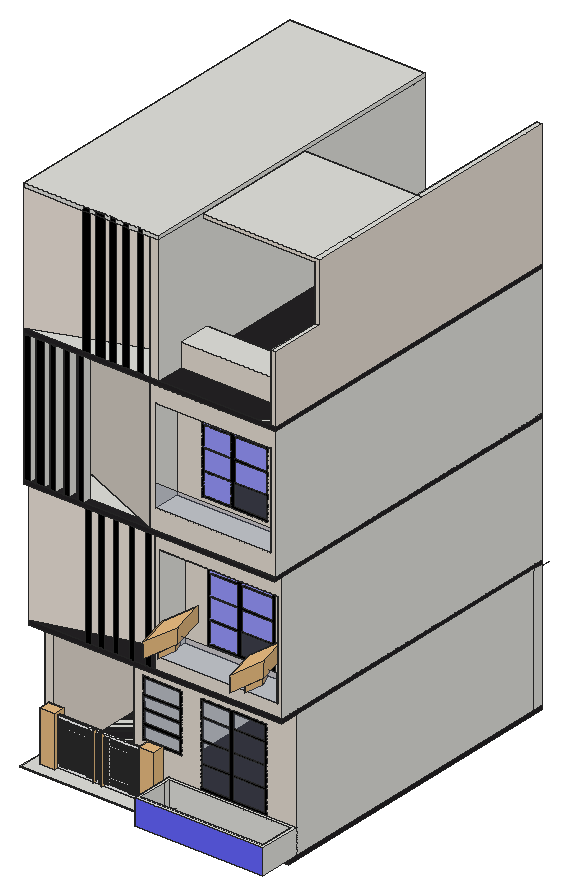
# SketchUp Ruby script. Lengths in inches.
U = 1.inch
M = Sketchup.active_model
def pt(a) = Geom::Point3d.new(a.map { |v| v * U })
def face(e, loops, mat)
  f = e.add_face(loops[0].map { |a| pt(a) })
  loops[1..].each { |l| e.add_face(l.map { |a| pt(a) }).erase! }
  f.material = f.back_material = mat if mat
  f
end
# faces: each face lists its corners as indices into pts; further lists are holes
def faces(e, pts, list, mat = nil) = list.each { |f| face(e, (f[0].is_a?(Array) ? f : [f]).map { |l| l.map { |i| pts[i] } }, mat) }
# xy, xz, yz: faces in a plane at the given z, y or x. An outline is a flat list of corners, or four numbers for a rectangle; further outlines are holes
def ring(l) = l.size == 4 ? [[l[0], l[1]], [l[2], l[1]], [l[2], l[3]], [l[0], l[3]]] : l.each_slice(2).to_a
def flat(e, list, mat, &to3) = list.each { |f| face(e, (f[0].is_a?(Array) ? f : [f]).map { |l| ring(l).map { |u, v| to3.(u, v) } }, mat) }
def xy(e, z, list, mat = nil) = flat(e, list, mat) { |x, y| [x, y, z] }
def xz(e, y, list, mat = nil) = flat(e, list, mat) { |x, z| [x, y, z] }
def yz(e, x, list, mat = nil) = flat(e, list, mat) { |y, z| [x, y, z] }
def lines(e, pts, list) = list.each { |a, b| e.add_line(pt(pts[a]), pt(pts[b])) }
# prism: a flat outline (further loops are holes) pulled along v
def prism(e, loops, v, mat = nil)
  f = face(e, loops, mat); d = Geom::Vector3d.new(v.map { |x| x * U })
  f.pushpull(f.normal.samedirection?(d) ? d.length : -d.length)
end
def box(e, o, s, mat = nil) = prism(e, [[o, [o[0] + s[0], o[1], o[2]], [o[0] + s[0], o[1] + s[1], o[2]], [o[0], o[1] + s[1], o[2]]]], [0, 0, s[2]], mat)
def at(x, y, z, deg = 0) = Geom::Transformation.translation(pt([x, y, z])) * Geom::Transformation.rotation(ORIGIN, Z_AXIS, deg.degrees)
def axes(o, x, y, z) = Geom::Transformation.new([*x, 0, *y, 0, *z, 0, *pt(o).to_a, 1])
def part(name) = M.definitions.add(name)
# library, detail: a bought-in or finely detailed component or shape, given as its bounding box
def library(name, o, s) = part(name).tap { |d| box(d.entities, o, s) }
def detail(e, o, s) = box(e.add_group.entities, o, s)
def put(e, d, t, mat = nil) = e.add_instance(d, t).tap { |i| i.material = mat if mat }
def group(e, t, mat = nil) = e.add_group.tap { |g| g.transformation = t; g.material = mat if mat }.entities
root = M.entities
M.materials.add("02 - Default").color = [196, 209, 187]
M.materials.add("02 - DefaultW").color = [91, 118, 29]
M.materials.add("04 - Default").color = [38, 38, 38]
M.materials.add("04 - DefaultW").color = [92, 55, 26]
M.materials.add("06 - Default").color = [255, 255, 255]
M.materials.add("07 - Default").color = [92, 55, 26]
M.materials.add("10 - Default").color = [62, 56, 39]
M.materials.add("Glass_Sky Reflection_01").color = [126, 138, 183]
M.materials["Glass_Sky Reflection_01"].alpha = 0.25
M.materials.add("I02_Moonlit_Azure").color = [153, 153, 255]
M.materials.add("I03_Bluebell_Mist").color = [101, 101, 255]
M.materials.add("M09_Shadow_Night").color = [0, 0, 0]
M.materials.add("Marble_01_1K").color = [230, 221, 211]
M.materials.add("Marble_07_1K").color = [36, 34, 36]
M.materials.add("Plywood_01_1K").color = [125, 96, 64]
M.materials.add("[Color_000]").color = [255, 255, 255]
M.materials.add("[Color_C20]").color = [102, 91, 81]
c1 = part("Horizontal gate slat")
xy(c1.entities,0,[[0.39,114.16,6.3,114.17]])
xy(c1.entities,0,[[0.39,0,6.3,114.16]],"[Color_C20]")
xy(c1.entities,0.39,[[0.39,0,0.79,114.17],[0.98,0,2.07,114.17],[2.36,0,3.2,114.17],[3.59,0,4.37,114.17],[4.56,0,5.71,114.17],
  [5.91,0,6.3,114.17]],"[Color_C20]")
xy(c1.entities,0.79,[[0.39,0,0.79,114.17],[0.98,0,2.07,114.17],[2.36,0,3.2,114.17],[3.59,0,4.37,114.17],[4.56,0,5.71,114.17],
  [5.91,0,6.3,114.17]],"[Color_C20]")
xy(c1.entities,0.99,[[1.13,0,1.21,114.16],[1.87,0,1.94,114.16],[2.61,0,2.68,114.16],[3.35,0,3.42,114.16],[4.08,0,4.16,114.16],
  [4.82,0,4.9,114.16],[5.5625,0,5.63,114.16],[6.3,0,6.37,114.16]],"[Color_C20]")
xy(c1.entities,1.18,[[0.39,114.16,3.35,114.17],[3.35,114.16,6.3,114.17]])
xy(c1.entities,1.18,[[0.39,0,1.13,114.16],[1.21,0,1.87,114.16],[1.94,0,2.61,114.16],[2.68,0,3.35,114.16],[3.42,0,4.08,114.16],
  [4.16,0,4.82,114.16],[4.9,0,5.5625,114.16],[5.63,0,6.3,114.16]],"[Color_C20]")
xz(c1.entities,0,[[[0.39,0,6.3,0,6.3,0.39,5.91,0.39,5.91,0.79,6.3,0.79,6.3,1.18,5.63,1.18,5.63,0.99,5.5625,0.99,5.5625,1.18,4.9,1.18,4.9,0.99,4.82,0.99,4.82,1.18,4.16,1.18,4.16,0.99,4.08,0.99,4.08,1.18,3.42,1.18,3.42,0.99,3.35,0.99,3.35,1.18,2.68,1.18,2.68,0.99,2.61,0.99,2.61,1.18,1.94,1.18,1.94,0.99,1.87,0.99,1.87,1.18,1.21,1.18,1.21,0.99,1.13,0.99,1.13,1.18,0.39,1.18,0.39,0.79,0.79,0.79,0.79,0.39,0.39,0.39],[4.56,0.39,5.71,0.79],[0.98,0.39,2.07,0.79],[2.36,0.39,3.2,0.79],[3.59,0.39,4.37,0.79]],[6.3,0.99,6.37,1.18]],"[Color_C20]")
xz(c1.entities,114.16,[[1.13,0.99,1.21,1.18],[1.87,0.99,1.94,1.18],[2.61,0.99,2.68,1.18],[3.35,0.99,3.42,1.18],[4.08,0.99,4.16,1.18],
  [4.82,0.99,4.9,1.18],[5.5625,0.99,5.63,1.18]],"[Color_C20]")
xz(c1.entities,114.17,[[[0.39,0,0.39,0.39,0.79,0.39,0.79,0.79,0.39,0.79,0.39,1.18,6.3,1.18,6.3,0.79,5.91,0.79,5.91,0.39,6.3,0.39,6.3,0],[4.56,0.39,5.71,0.79],[0.98,0.39,2.07,0.79],[2.36,0.39,3.2,0.79],[3.59,0.39,4.37,0.79]]],"[Color_C20]")
yz(c1.entities,0.39,[[114.16,0,114.17,0.39],[114.16,0.79,114.17,1.18]])
yz(c1.entities,0.39,[[0,0,114.16,0.39],[0,0.79,114.16,1.18]],"[Color_C20]")
yz(c1.entities,0.79,[[0,0.39,114.17,0.79]],"[Color_C20]")
yz(c1.entities,0.98,[[0,0.39,114.17,0.79]],"[Color_C20]")
yz(c1.entities,1.13,[[0,0.99,114.16,1.18]],"[Color_C20]")
yz(c1.entities,1.21,[[0,0.99,114.16,1.18]],"[Color_C20]")
yz(c1.entities,1.87,[[0,0.99,114.16,1.18]],"[Color_C20]")
yz(c1.entities,1.94,[[0,0.99,114.16,1.18]],"[Color_C20]")
yz(c1.entities,2.07,[[0,0.39,114.17,0.79]],"[Color_C20]")
yz(c1.entities,2.36,[[0,0.39,114.17,0.79]],"[Color_C20]")
yz(c1.entities,2.61,[[0,0.99,114.16,1.18]],"[Color_C20]")
yz(c1.entities,2.68,[[0,0.99,114.16,1.18]],"[Color_C20]")
yz(c1.entities,3.2,[[0,0.39,114.17,0.79]],"[Color_C20]")
yz(c1.entities,3.35,[[0,0.99,114.16,1.18]],"[Color_C20]")
yz(c1.entities,3.42,[[0,0.99,114.16,1.18]],"[Color_C20]")
yz(c1.entities,3.59,[[0,0.39,114.17,0.79]],"[Color_C20]")
yz(c1.entities,4.08,[[0,0.99,114.16,1.18]],"[Color_C20]")
yz(c1.entities,4.16,[[0,0.99,114.16,1.18]],"[Color_C20]")
yz(c1.entities,4.37,[[0,0.39,114.17,0.79]],"[Color_C20]")
yz(c1.entities,4.56,[[0,0.39,114.17,0.79]],"[Color_C20]")
yz(c1.entities,4.82,[[0,0.99,114.16,1.18]],"[Color_C20]")
yz(c1.entities,4.9,[[0,0.99,114.16,1.18]],"[Color_C20]")
yz(c1.entities,5.5625,[[0,0.99,114.16,1.18]],"[Color_C20]")
yz(c1.entities,5.63,[[0,0.99,114.16,1.18]],"[Color_C20]")
yz(c1.entities,5.71,[[0,0.39,114.17,0.79]],"[Color_C20]")
yz(c1.entities,5.91,[[0,0.39,114.17,0.79]],"[Color_C20]")
yz(c1.entities,6.3,[[114.16,0,114.17,0.39],[114.16,0.79,114.17,1.18]])
yz(c1.entities,6.3,[[0,0,114.16,0.39],[0,0.79,114.16,0.99],[0,0.99,114.16,1.18]],"[Color_C20]")
yz(c1.entities,6.37,[[0,0.99,114.16,1.18]],"[Color_C20]")
p = [[0,0,0],[0.39,0,0]]
lines(c1.entities,p,[[0,1]])
c2 = part("Vertical gate panel")
put(c2.entities,c1,axes([0,1.18,0],[3.67755,0,0],[0,0,2.40086],[0,-1,0]))
put(c2.entities,c1,axes([21.72,1.18,0],[3.67755,0,0],[0,0,2.40086],[0,-1,0]))
c3 = library("Gate pull handle",[-0.01,0,0],[1.26,2.875,48])
c4 = part("Slatted gate assembly")
xy(c4.entities,0,[[553.15,18.86,552.64,18.92,552.18,19.1,551.78,19.39,551.47,19.76,551.27,20.2,551.21,20.67,551.27,21.13,551.47,21.57,551.78,21.94,552.18,22.23,552.64,22.41,553.15,22.47,553.65,22.41,554.11,22.23,554.52,21.94,554.82,21.57,555.02,21.13,555.08,20.67,555.02,20.2,554.82,19.76,554.52,19.39,554.11,19.1,553.65,18.92],[12.73,19.29,12.23,19.35,11.76,19.55,11.36,19.85,11.05,20.25,10.86,20.72,10.79,21.22,10.86,21.72,11.05,22.19,11.36,22.59,11.76,22.9,12.23,23.09,12.73,23.16,13.23,23.09,13.7,22.9,14.1,22.59,14.41,22.19,14.6,21.72,14.67,21.22,14.6,20.72,14.41,20.25,14.1,19.85,13.7,19.55,13.23,19.35]])
xy(c4.entities,5.93,[[[4.54,12.88,282.375,27.63],[12.73,19.29,13.23,19.35,13.7,19.55,14.1,19.85,14.41,20.25,14.6,20.72,14.67,21.22,14.6,21.72,14.41,22.19,14.1,22.59,13.7,22.9,13.23,23.09,12.73,23.16,12.23,23.09,11.76,22.9,11.36,22.59,11.05,22.19,10.86,21.72,10.79,21.22,10.86,20.72,11.05,20.25,11.36,19.85,11.76,19.55,12.23,19.35]],[[283.5,12.88,556.09,26.65],[553.15,18.86,553.65,18.92,554.11,19.1,554.52,19.39,554.82,19.76,555.02,20.2,555.08,20.67,555.02,21.13,554.82,21.57,554.52,21.94,554.11,22.23,553.65,22.41,553.15,22.47,552.64,22.41,552.18,22.23,551.78,21.94,551.47,21.57,551.27,21.13,551.21,20.67,551.27,20.2,551.47,19.76,551.78,19.39,552.18,19.1,552.64,18.92]]],"[Color_000]")
xy(c4.entities,21.29,[[73.46,12.88,80.01,15.32],[80.01,12.88,217.27,15.32],[217.27,12.88,223.83,15.32],[342.04,12.88,348.6,15.16],[348.6,12.88,485.86,15.16],
  [485.86,12.88,492.42,15.16]])
xy(c4.entities,21.29,[[30.27,12.88,51.87,27.63],[51.87,12.88,73.46,27.63],[223.83,12.88,267.01,15.32],[298.86,12.88,342.04,15.16],[492.42,12.88,514.01,26.65],
  [514.01,12.88,535.6,26.65],[298.86,15.16,342.04,26.65],[348.6,15.16,485.86,26.65],[80.01,15.32,217.27,27.63],[223.83,15.32,267.01,27.63]],"[Color_000]")
xy(c4.entities,27.1,[[4.54,12.88,14.91,27.63],[550.96,12.88,556.09,26.65]],"[Color_000]")
xy(c4.entities,64.47,[[80.01,12.88,217.27,27.63],[348.6,12.88,485.86,26.65]],"[Color_000]")
xy(c4.entities,71.03,[[80.01,12.88,217.27,27.63],[348.6,12.88,485.86,26.65]],"[Color_000]")
xy(c4.entities,245.66,[[80.01,12.88,217.27,27.63],[348.6,12.88,485.86,26.65]],"[Color_000]")
xy(c4.entities,252.22,[[80.01,12.88,217.27,27.63],[348.6,12.88,485.86,26.65]],"[Color_000]")
xy(c4.entities,253.46,[[550.96,17.74,555.84,22.93],[10.04,18.09,14.91,23.65]],"[Color_000]")
xy(c4.entities,263.88,[[550.96,17.74,555.84,22.93],[10.04,18.09,14.91,23.65]],"[Color_000]")
xy(c4.entities,264.34,[[550.96,17.74,555.84,22.93],[555.84,17.74,565.875,22.93],[0,18.09,10.04,23.65],[10.04,18.09,14.91,23.65]],"[Color_000]")
xy(c4.entities,267.5,[[550.96,17.74,555.84,22.93],[555.84,17.74,565.875,22.93],[0,18.09,10.04,23.65],[10.04,18.09,14.91,23.65]],"[Color_000]")
xy(c4.entities,268.01,[[550.96,17.74,555.84,22.93],[10.04,18.09,14.91,23.65]],"[Color_000]")
xy(c4.entities,278.02,[[550.96,17.74,555.84,22.93],[10.04,18.09,14.91,23.65]],"[Color_000]")
xy(c4.entities,295.4,[[30.27,12.88,51.87,27.63],[51.87,12.88,73.46,27.63],[80.01,12.88,217.27,27.63],[223.83,12.88,267.01,27.63],[298.86,12.88,342.04,26.65],
  [348.6,12.88,485.86,26.65],[492.42,12.88,514.01,26.65],[514.01,12.88,535.6,26.65]],"[Color_000]")
xy(c4.entities,310.76,[[14.91,12.88,282.375,27.63],[283.5,12.88,550.96,26.65]],"[Color_000]")
xz(c4.entities,12.88,[[[4.54,5.93,282.375,5.93,282.375,310.76,14.91,310.76,14.91,27.1,4.54,27.1],[30.27,21.29,267.01,295.4]],[[283.5,5.93,556.09,5.93,556.09,27.1,550.96,27.1,550.96,310.76,283.5,310.76],[298.86,21.29,535.6,295.4]],[73.46,21.29,80.01,64.47],[217.27,21.29,223.83,64.47],[342.04,21.29,348.6,64.47],
  [485.86,21.29,492.42,64.47],[73.46,64.47,223.83,64.47,223.83,252.22,73.46,252.22,73.46,245.66,217.27,245.66,217.27,71.03,80.01,71.03,80.01,245.66,73.46,245.66],[342.04,64.47,492.42,64.47,492.42,245.66,485.86,245.66,485.86,71.03,348.6,71.03,348.6,245.66,492.42,245.66,492.42,252.22,342.04,252.22],[73.46,252.22,80.01,295.4],[217.27,252.22,223.83,295.4],
  [342.04,252.22,348.6,295.4],[485.86,252.22,492.42,295.4]],"[Color_000]")
xz(c4.entities,17.74,[[550.96,253.46,555.84,263.88],[550.96,264.34,565.875,267.5],[550.96,268.01,555.84,278.02]],"[Color_000]")
xz(c4.entities,18.09,[[10.04,253.46,14.91,263.88],[0,264.34,14.91,267.5],[10.04,268.01,14.91,278.02]],"[Color_000]")
xz(c4.entities,22.93,[[550.96,253.46,555.84,263.88],[550.96,264.34,555.84,265.59],[555.84,264.34,555.84,265.59,550.96,265.59,550.96,267.5,565.875,267.5,565.875,264.34],[550.96,268.01,555.84,278.02]],"[Color_000]")
xz(c4.entities,23.65,[[10.04,253.46,14.91,263.88],[0,264.34,0,267.5,14.91,267.5,14.91,265.59,10.04,265.59,10.04,264.34],[10.04,264.34,14.91,265.59],[10.04,268.01,14.91,278.02]],"[Color_000]")
xz(c4.entities,26.65,[[[283.5,5.93,283.5,310.76,550.96,310.76,550.96,27.1,556.09,27.1,556.09,5.93],[348.6,71.03,485.86,245.66],[492.42,21.29,535.6,295.4],[298.86,21.29,342.04,295.4],[348.6,252.22,485.86,295.4],[348.6,21.29,485.86,64.47]]],"[Color_000]")
xz(c4.entities,27.63,[[[4.54,5.93,4.54,27.1,14.91,27.1,14.91,310.76,282.375,310.76,282.375,5.93],[80.01,71.03,217.27,245.66],[30.27,21.29,73.46,295.4],[223.83,21.29,267.01,295.4],[80.01,252.22,217.27,295.4],[80.01,21.29,217.27,64.47]]],"[Color_000]")
yz(c4.entities,0,[[18.09,264.34,23.65,267.5]],"[Color_000]")
yz(c4.entities,4.54,[[12.88,5.93,27.63,27.1]],"[Color_000]")
yz(c4.entities,10.04,[[18.09,253.46,23.65,263.88],[18.09,268.01,23.65,278.02]],"[Color_000]")
yz(c4.entities,14.91,[[[12.88,27.1,27.63,310.76],[18.09,253.46,23.65,263.88],[18.09,268.01,23.65,278.02],[18.09,264.34,23.65,267.5]]],"[Color_000]")
yz(c4.entities,30.27,[[12.88,21.29,27.63,295.4]],"[Color_000]")
yz(c4.entities,73.46,[[12.88,21.29,27.63,64.47],[12.88,64.47,27.63,245.66],[12.88,245.66,27.63,252.22],[12.88,252.22,27.63,295.4]],"[Color_000]")
yz(c4.entities,80.01,[[12.88,21.29,27.63,64.47],[12.88,71.03,27.63,245.66],[12.88,252.22,27.63,295.4]],"[Color_000]")
yz(c4.entities,217.27,[[12.88,21.29,27.63,64.47],[12.88,71.03,27.63,245.66],[12.88,252.22,27.63,295.4]],"[Color_000]")
yz(c4.entities,223.83,[[12.88,21.29,27.63,64.47],[12.88,64.47,27.63,252.22],[12.88,252.22,27.63,295.4]],"[Color_000]")
yz(c4.entities,267.01,[[12.88,21.29,27.63,295.4]],"[Color_000]")
yz(c4.entities,282.375,[[12.88,5.93,27.63,310.76]],"[Color_000]")
yz(c4.entities,283.5,[[12.88,5.93,26.65,310.76]],"[Color_000]")
yz(c4.entities,298.86,[[12.88,21.29,26.65,295.4]],"[Color_000]")
yz(c4.entities,342.04,[[12.88,21.29,26.65,64.47],[12.88,64.47,26.65,252.22],[12.88,252.22,26.65,295.4]],"[Color_000]")
yz(c4.entities,348.6,[[12.88,21.29,26.65,64.47],[12.88,71.03,26.65,245.66],[12.88,252.22,26.65,295.4]],"[Color_000]")
yz(c4.entities,485.86,[[12.88,21.29,26.65,64.47],[12.88,71.03,26.65,245.66],[12.88,252.22,26.65,295.4]],"[Color_000]")
yz(c4.entities,492.42,[[12.88,21.29,26.65,64.47],[12.88,64.47,26.65,245.66],[12.88,245.66,26.65,252.22],[12.88,252.22,26.65,295.4]],"[Color_000]")
yz(c4.entities,535.6,[[12.88,21.29,26.65,295.4]],"[Color_000]")
yz(c4.entities,550.96,[[[12.88,27.1,26.65,310.76],[17.74,253.46,17.74,263.88,22.93,263.88,22.93,264.34,17.74,264.34,17.74,267.5,22.93,267.5,22.93,253.46],[17.74,268.01,22.93,278.02]]],"[Color_000]")
yz(c4.entities,555.84,[[17.74,253.46,22.93,263.88],[17.74,268.01,22.93,278.02]],"[Color_000]")
yz(c4.entities,556.09,[[12.88,5.93,26.65,27.1]],"[Color_000]")
p = [[552.64,18.92,5.93],[552.18,19.1,5.93],[552.18,19.1,0],[552.64,18.92,0],[553.15,18.86,5.93],[553.15,18.86,0],
  [553.65,18.92,5.93],[553.65,18.92,0],[554.11,19.1,5.93],[554.11,19.1,0],[551.78,19.39,5.93],[551.78,19.39,0],
  [554.52,19.39,5.93],[554.52,19.39,0],[12.73,19.29,5.93],[12.23,19.35,5.93],[12.23,19.35,0],[12.73,19.29,0],
  [13.23,19.35,5.93],[13.23,19.35,0],[11.76,19.55,5.93],[11.76,19.55,0],[13.7,19.55,5.93],[13.7,19.55,0],
  [551.47,19.76,5.93],[551.47,19.76,0],[554.82,19.76,5.93],[554.82,19.76,0],[11.36,19.85,5.93],[11.36,19.85,0],
  [14.1,19.85,5.93],[14.1,19.85,0],[551.27,20.2,5.93],[551.27,20.2,0],[555.02,20.2,5.93],[555.02,20.2,0],
  [11.05,20.25,5.93],[11.05,20.25,0],[14.41,20.25,5.93],[14.41,20.25,0],[551.21,20.67,5.93],[551.21,20.67,0],
  [555.08,20.67,5.93],[555.08,20.67,0],[10.86,20.72,5.93],[10.86,20.72,0],[14.6,20.72,5.93],[14.6,20.72,0],
  [10.79,21.22,5.93],[10.79,21.22,0],[14.67,21.22,5.93],[14.67,21.22,0],[551.27,21.13,5.93],[551.27,21.13,0],
  [555.02,21.13,5.93],[555.02,21.13,0],[551.47,21.57,5.93],[551.47,21.57,0],[554.82,21.57,5.93],[554.82,21.57,0],
  [10.86,21.72,5.93],[10.86,21.72,0],[14.6,21.72,5.93],[14.6,21.72,0],[551.78,21.94,5.93],[551.78,21.94,0],
  [554.52,21.94,5.93],[554.52,21.94,0],[11.05,22.19,5.93],[11.05,22.19,0],[14.41,22.19,5.93],[14.41,22.19,0],
  [552.18,22.23,5.93],[552.18,22.23,0],[554.11,22.23,5.93],[554.11,22.23,0],[11.36,22.59,5.93],[11.36,22.59,0],
  [14.1,22.59,5.93],[14.1,22.59,0],[552.64,22.41,5.93],[552.64,22.41,0],[553.65,22.41,5.93],[553.65,22.41,0],
  [553.15,22.47,5.93],[553.15,22.47,0],[11.76,22.9,5.93],[11.76,22.9,0],[13.7,22.9,5.93],[13.7,22.9,0],
  [12.23,23.09,5.93],[12.23,23.09,0],[13.23,23.09,5.93],[13.23,23.09,0],[12.73,23.16,5.93],[12.73,23.16,0],
  [495.13,15.16,21.29],[492.42,15.16,21.29],[505.99,15.16,295.37],[348.6,15.16,295.37],[485.84,15.16,253.84],[485.84,15.16,71.03],
  [59.88,15.32,295.37],[217.27,15.32,295.37],[70.74,15.32,21.29],[73.46,15.32,21.29],[80.03,15.32,253.84],[80.03,15.32,71.03],
  [282.375,12.88,5.93],[283.5,12.88,5.93],[14.91,23.65,264.34],[14.91,23.65,263.88]]
faces(c4.entities,p,[[0,1,2,3],[4,0,3,5],[6,4,5,7],[8,6,7,9],[1,10,11,2],[12,8,9,13],[14,15,16,17],[18,14,17,19],
  [15,20,21,16],[22,18,19,23],[10,24,25,11],[26,12,13,27],[20,28,29,21],[30,22,23,31],[24,32,33,25],[34,26,27,35],
  [28,36,37,29],[38,30,31,39],[32,40,41,33],[42,34,35,43],[36,44,45,37],[46,38,39,47],[44,48,49,45],[50,46,47,51],
  [40,52,53,41],[54,42,43,55],[52,56,57,53],[58,54,55,59],[48,60,61,49],[62,50,51,63],[56,64,65,57],[66,58,59,67],
  [60,68,69,61],[70,62,63,71],[64,72,73,65],[74,66,67,75],[68,76,77,69],[78,70,71,79],[72,80,81,73],[82,74,75,83],
  [80,84,85,81],[84,82,83,85],[76,86,87,77],[88,78,79,89],[86,90,91,87],[92,88,89,93],[90,94,95,91],[94,92,93,95]],"[Color_000]")
lines(c4.entities,p,[[96,97],[98,99],[100,101],[102,103],[104,105],[106,107],[108,109],[110,111]])
put(c4.entities,c2,axes([217.26,15.32,19.8125],[0,0,1.01983],[0,1,0],[-0.50074,0,0]))
put(c4.entities,c1,axes([222.13,16.5,21.29],[3.67755,0,0],[0,0,2.40086],[0,-1,0]))
put(c4.entities,c2,axes([217.29,15.32,113.92],[0,0,0.9999],[0,1,0],[-0.50074,0,0]))
put(c4.entities,c2,axes([217.27,15.32,200.78],[0,0,0.9999],[0,1,0],[-0.50074,0,0]))
put(c4.entities,c2,axes([217.29,15.32,70.49],[0,0,0.9999],[0,1,0],[-0.50074,0,0]))
put(c4.entities,c2,axes([217.27,15.32,249.59],[0,0,1.01983],[0,1,0],[-0.50074,0,0]))
put(c4.entities,c2,axes([217.27,15.32,157.35],[0,0,0.9999],[0,1,0],[-0.50074,0,0]))
put(c4.entities,c3,axes([253.77,0,7.15],[4.3,0,0],[0,4.47827,0],[0,0,6.3253]))
put(c4.entities,c1,axes([322.03,16.26,21.29],[-3.67755,0,0],[0,0,2.40086],[0,-0.93319,0]))
put(c4.entities,c1,axes([28.57,16.5,21.29],[3.67755,0,0],[0,0,2.40086],[0,-1,0]))
put(c4.entities,c1,axes([243.85,16.5,21.29],[3.67755,0,0],[0,0,2.40086],[0,-1,0]))
put(c4.entities,c1,axes([50.29,16.5,21.29],[3.67755,0,0],[0,0,2.40086],[0,-1,0]))
put(c4.entities,c2,axes([348.62,15.16,19.8125],[0,0,1.01983],[0,0.93319,0],[0.50074,0,0]))
put(c4.entities,c2,axes([348.6,15.16,249.59],[0,0,1.01983],[0,0.93319,0],[0.50074,0,0]))
put(c4.entities,c2,axes([348.6,15.16,200.78],[0,0,0.9999],[0,0.93319,0],[0.50074,0,0]))
put(c4.entities,c1,axes([537.3,16.26,21.29],[-3.67755,0,0],[0,0,2.40086],[0,-0.93319,0]))
put(c4.entities,c1,axes([515.58,16.26,21.29],[-3.67755,0,0],[0,0,2.40086],[0,-0.93319,0]))
put(c4.entities,c3,axes([312.11,0.86,7.15],[-4.3,0,0],[0,4.17906,0],[0,0,6.3253]))
put(c4.entities,c2,axes([348.58,15.16,113.92],[0,0,0.9999],[0,0.93319,0],[0.50074,0,0]))
put(c4.entities,c2,axes([348.6,15.16,157.35],[0,0,0.9999],[0,0.93319,0],[0.50074,0,0]))
put(c4.entities,c2,axes([348.58,15.16,70.49],[0,0,0.9999],[0,0.93319,0],[0.50074,0,0]))
put(c4.entities,c1,axes([343.75,16.26,21.29],[-3.67755,0,0],[0,0,2.40086],[0,-0.93319,0]))
c5 = library("Capped gate post",[0,0,0],[97.06,71.13,326.45])
c6 = part("T gate")
box(c6.entities,[-71.08,-89.97,-2.875],[892.43,222.56,2.875])
put(c6.entities,c4,at(79.05,-4.33,0))
put(c6.entities,c5,at(-9.01,-9.01,0))
put(c6.entities,c5,axes([732.98,-9.01,0],[-1,0,0],[0,1,0],[0,0,1]))
c7 = library("MONSTERA_Defintion",[-100.72,-132.16,0],[226.75,232.88,1000])
c8 = library("MONSTERA_Defintion1",[-382.23,-503.1,29.34],[811.96,1000,773.77])
c9 = library("POT_Defintion",[-467.71,-467.71,0],[935.42,935.42,1000])
c10 = library("POT_Defintion6",[-504.36,-499.05,1069.94],[1000,1000,51.81])
c11 = library("TABLE_Defintion5",[-349.98,-500,-99.29],[912.18,1000,162.92])
c12 = library("TABLE_Defintion3",[-282.7,-491.23,-690.5],[848.82,1000,669.35])
c13 = library("TABLE_Defintion",[-354.24,-500,-9.27],[914.7,1000,77.28])
c14 = part("Monstera Plant 50")
g1 = group(c14.entities,at(0,0,0))
g2 = group(g1,at(0,0,0))
put(g2,c7,axes([-70.21,316.62,1332.52],[0.60525,0.72131,0],[-0.72131,0.60525,0],[0,0,0.92363]),"02 - DefaultW")
put(g2,c8,axes([-70.21,316.62,1332.52],[2.09136,2.49238,0],[-2.49238,2.09136,0],[0,0,3.1915]),"02 - Default")
g3 = group(c14.entities,at(0,0,0))
g4 = group(g3,at(0,0,0))
put(g4,c9,axes([-63.73,311.08,962.21],[0.47902,0.57088,0],[-0.57088,0.47902,0],[0,0,0.69328]),"04 - Default")
put(g4,c10,axes([-63.73,311.08,962.21],[0.41695,0.4969,0],[-0.4969,0.41695,0],[0,0,0.60345]),"10 - Default")
g5 = group(c14.entities,at(0,0,0))
g6 = group(g5,at(0,0,0))
put(g6,c11,axes([-8.95,303.3125,886.6],[1.07163,-0.6187,0],[0.6187,1.07163,0],[0,0,1.23741]),"04 - DefaultW")
put(g6,c12,axes([-8.95,303.3125,886.6],[1.11435,-0.64337,0],[0.64337,1.11435,0],[0,0,1.28674]),"07 - Default")
put(g6,c13,axes([-8.95,303.3125,886.6],[1.10303,-0.63684,0],[0.63684,1.10303,0],[0,0,1.27367]),"06 - Default")
box(root,[4.4,65.84,252],[119.53,265.15,123.85])
xy(root,252,[[4.4,14.07,10.92,21.73],[15.95,14.07,24.54,21.73],[29.43,14.07,35.24,21.73],[42.21,14.07,48.17,21.73],[56.09,14.07,61.4375,21.73]])
xy(root,375.85,[[4.4,14.07,10.92,21.73],[15.95,14.07,24.54,21.73],[29.43,14.07,35.24,21.73],[42.21,14.07,48.17,21.73],[56.09,14.07,61.4375,21.73]])
xy(root,499.85,[[3.59,15.21,132.09,330.99]])
xy(root,503.85,[[3.59,15.21,132.09,330.99]])
xz(root,14.07,[[4.4,252,10.92,375.85],[15.95,252,24.54,375.85],[29.43,252,35.24,375.85],[42.21,252,48.17,375.85],[56.09,252,61.4375,375.85]],"M09_Shadow_Night")
xz(root,14.85,[[129.9,271.25,238.84,292.23]],"Glass_Sky Reflection_01")
xz(root,15.21,[[3.59,499.85,60.1,499.85,60.1,503.69,66.61,503.69,66.61,499.85,71.64,499.85,71.64,503.69,80.24,503.69,80.24,499.85,85.125,499.85,85.125,503.69,90.9375,503.69,90.9375,499.85,97.91,499.85,97.91,503.69,103.86,503.69,103.86,499.85,111.79,499.85,111.79,503.69,117.13,503.69,117.13,499.85,132.09,499.85,132.09,503.85,3.59,503.85]])
xz(root,15.21,[[60.1,379.85,66.61,499.85],[71.64,379.85,80.24,499.85],[85.125,379.85,90.9375,499.85],[97.91,379.85,103.86,499.85],[111.79,379.85,117.13,499.85],
  [60.1,499.85,66.61,503.69],[71.64,499.85,80.24,503.69],[85.125,499.85,90.9375,503.69],[97.91,499.85,103.86,503.69],[111.79,499.85,117.13,503.69]],"M09_Shadow_Night")
xz(root,21.73,[[4.4,252,10.92,375.85],[15.95,252,24.54,375.85],[29.43,252,35.24,375.85],[42.21,252,48.17,375.85],[56.09,252,61.4375,375.85]])
xz(root,21.73,[[128.14,139.58,239.53,165.69]],"Glass_Sky Reflection_01")
xz(root,21.73,[[57.61,128,62.09,248],[70.13,128,74.6,248],[83.67,128,88.15,248],[98.91,128,103.39,248],[114.7,128,119.17,248]],"M09_Shadow_Night")
xz(root,330.99,[[3.59,499.85,132.09,503.85]])
yz(root,3.59,[[15.21,499.85,330.99,503.85]])
yz(root,4.4,[[14.07,252,21.73,375.85]])
yz(root,10.92,[[14.07,252,21.73,375.85]])
yz(root,15.95,[[14.07,252,21.73,375.85]])
yz(root,24.54,[[14.07,252,21.73,375.85]])
yz(root,29.43,[[14.07,252,21.73,375.85]])
yz(root,35.24,[[14.07,252,21.73,375.85]])
yz(root,42.21,[[14.07,252,21.73,375.85]])
yz(root,48.17,[[14.07,252,21.73,375.85]])
yz(root,56.09,[[14.07,252,21.73,375.85]])
yz(root,61.4375,[[14.07,252,21.73,375.85]])
yz(root,132.09,[[15.21,499.85,330.99,503.85]])
p = [[242.32,341.6,121.84],[242.32,332.6,121.84],[244.97,330.49,254.625],[244.97,321.49,254.625]]
lines(root,p,[[0,1],[2,3]])
put(root,c6,axes([10.43,28.51,5.21],[0.14671,0,0],[0,0.14671,0],[0,0,0.14671]))
put(root,c14,axes([224.375,10.24,153.45],[0.00356,0,0],[0,0.01663,0],[0,0,0.00573]))
put(root,c14,axes([142.31,10.24,153.45],[0.00356,0,0],[0,0.01663,0],[0,0,0.00573]))
g7 = group(root,at(3.45,30.99,0),"Marble_07_1K")
box(g7,[0,0,0],[240,300,4])
g8 = group(root,at(3.45,0,4))
xy(g8,0,[[121.23,3.41,236.59,36.58],[0,30.99,117.82,30.99,117.82,39.99,9,39.99,9,40.37,0,40.37],[9,39.99,85.4375,321.99]])
xy(g8,23.72,[[[117.82,0,240,39.99],[121.23,3.41,236.59,36.58]]])
xy(g8,120,[[85.4375,39.99,240,321.99],[0,40.37,9,40.37,9,321.99,240,321.99,240,330.99,0,330.99]])
xz(g8,0,[[117.82,0,240,23.72]],"I03_Bluebell_Mist")
xz(g8,3.41,[[121.23,0,236.59,23.72]])
xz(g8,36.58,[[121.23,0,236.59,23.72]])
xz(g8,39.99,[[150.3125,25.59,176.48,45.57],[180.12,25.59,209.93,45.57],[150.3125,46.63,176.48,65.55],[180.12,46.63,209.93,65.55],[94.97,48.46,128.64,59.16],
  [94.97,61.51,128.64,73.18],[150.3125,66.61,176.48,85.52],[180.12,66.61,209.93,85.52],[94.97,74.56,128.64,74.56,128.64,76.06,128.58,85.05,94.92,85.05,94.97,76.06],[150.3125,86.59,176.48,99.89],
  [180.12,86.59,209.93,99.89],[94.95,86.7,128.61,86.7,128.64,88.35,128.64,99.88,94.97,99.88,94.97,88.35]],"Glass_Sky Reflection_01")
xz(g8,39.99,[[[148.44,23.72,211.79,101.76],[180.12,25.59,209.93,45.57],[180.12,46.63,209.93,65.55],[180.12,66.61,209.93,85.52],[150.3125,25.59,176.48,45.57],[150.3125,66.61,176.48,85.52],[150.3125,46.63,176.48,65.55],[180.12,86.59,209.93,99.89],[150.3125,86.59,176.48,99.89]],[[93.09,46.58,130.52,101.76],[94.95,86.7,94.97,88.35,94.97,99.88,128.64,99.88,128.64,88.35,128.61,86.7],[94.97,61.51,128.64,73.18],[94.97,48.46,128.64,59.16],[94.97,74.56,94.97,76.06,94.92,85.05,128.58,85.05,128.64,76.06,128.64,74.56]]],"M09_Shadow_Night")
xz(g8,39.99,[[[85.4375,0,117.82,0,117.82,23.72,148.44,23.72,148.44,101.76,211.79,101.76,211.79,23.72,240,23.72,240,120,85.4375,120],[93.09,46.58,130.52,101.76]]],"Marble_01_1K")
xz(g8,40.37,[[0,0,9,120]],"Marble_01_1K")
xz(g8,321.99,[[9,0,85.4375,120]],"Marble_01_1K")
xz(g8,330.99,[[0,0,240,120]])
yz(g8,0,[[40.37,0,330.99,120]])
yz(g8,9,[[40.37,0,321.99,120]],"Marble_01_1K")
yz(g8,85.4375,[[39.99,0,321.99,120]])
yz(g8,117.82,[[0,0,30.99,23.72],[30.99,0,39.99,23.72]])
yz(g8,121.23,[[3.41,0,30.99,23.72],[30.99,0,36.58,23.72]])
yz(g8,236.59,[[3.41,0,36.58,23.72]])
yz(g8,240,[[0,0,39.99,23.72],[39.99,0,321.99,120],[321.99,0,330.99,120]])
g9 = group(root,at(3.45,21.73,124),"Marble_07_1K")
box(g9,[0,0,0],[240,309.26,4])
g10 = group(root,at(3.45,21.73,128))
xy(g10,0,[[120,0,120,35.15,0.96,35.15,0.96,309.26,240,309.26,240,0]])
xy(g10,11.58,[[124.69,0,236.09,28.87]])
xy(g10,104.03,[[124.69,0,236.09,28.87]])
xy(g10,120,[[120,0,240,0,240,309.26,0.96,309.26,0.96,35.15,120,35.15]])
xz(g10,0,[[[120,0,240,120],[124.69,11.58,236.09,104.03]]],"Marble_01_1K")
xz(g10,28.87,[[179,19.44,208.81,39.41]],"Glass_Sky Reflection_01")
xz(g10,28.87,[[149.19,19.44,175.35,39.41],[149.19,40.48,175.35,59.39],[179,40.48,208.81,59.39],[149.19,60.46,175.35,79.37],[179,60.46,208.81,79.37],
  [149.19,80.43,175.35,93.73],[179,80.43,208.81,93.73]],"I02_Moonlit_Azure")
xz(g10,28.87,[[147.32,17.57,149.19,17.57,149.19,93.73,210.67,93.73,210.67,95.6,147.32,95.6],[[149.19,17.57,210.67,17.57,210.67,93.73,208.81,93.73,208.81,80.43,179,80.43,179,93.73,175.35,93.73,175.35,80.43,149.19,80.43,149.19,79.37,175.35,79.37,175.35,60.46,149.19,60.46,149.19,59.39,175.35,59.39,175.35,40.48,149.19,40.48,149.19,39.41,175.35,39.41,175.35,19.44,149.19,19.44],[179,19.44,208.81,39.41],[179,60.46,208.81,79.37],[179,40.48,208.81,59.39]]],"M09_Shadow_Night")
xz(g10,28.87,[[[124.69,11.58,236.09,104.03],[147.32,19.44,210.67,95.6],[147.32,17.57,147.32,95.6,210.67,95.6,210.67,93.73,149.19,93.73,149.19,17.57]]],"Marble_01_1K")
xz(g10,35.15,[[0.96,0,120,120]])
xz(g10,309.26,[[0.96,0,240,120]])
yz(g10,0.96,[[35.15,0,309.26,120]])
yz(g10,120,[[0,0,35.15,120]])
yz(g10,124.69,[[0,11.58,28.87,104.03]])
yz(g10,236.09,[[0,11.58,28.87,104.03]])
yz(g10,240,[[0,0,309.26,120]])
p = [[0,0,0],[120,35.15,0],[120,35.15,120],[0,0,120],[0,309.26,0],[0.96,309.26,0]]
faces(g10,p,[[0,1,2,3]],"Marble_01_1K")
lines(g10,p,[[4,5]])
g11 = group(root,at(4.4,21.73,248),"Marble_07_1K")
box(g11,[0,-7.66,0],[239.04,316.92,4])
g12 = group(root,at(4.4,14.85,252))
xy(g12,0,[[119.52,0,119.52,6.89,103.38,6.89],[119.52,0,239.04,6.89],[0,6.89,103.38,6.89,0,50.99],[103.38,6.89,119.52,6.89,119.52,316.14,0,316.14,0,50.99]])
xy(g12,19.25,[[125.5,0,234.4375,24.64]])
xy(g12,108.61,[[125.5,0,234.4375,24.64]])
xy(g12,123.85,[[119.52,0,239.04,316.14]])
xz(g12,0,[[[119.52,0,239.04,123.85],[125.5,19.25,234.4375,108.61]]],"Marble_01_1K")
xz(g12,24.64,[[180.6875,28.22,210.49,48.19]],"Glass_Sky Reflection_01")
xz(g12,24.64,[[150.88,28.22,177.04,48.19],[150.88,49.26,177.04,68.17],[180.6875,49.26,210.49,68.17],[150.88,69.24,177.04,88.15],[180.6875,69.24,210.49,88.15],
  [150.88,89.22,177.04,102.52],[180.6875,89.22,210.49,102.52]],"I02_Moonlit_Azure")
xz(g12,24.64,[[149.01,26.35,150.88,26.35,150.88,102.52,212.36,102.52,212.36,104.38,149.01,104.38],[[150.88,26.35,212.36,26.35,212.36,102.52,210.49,102.52,210.49,89.22,180.6875,89.22,180.6875,102.52,177.04,102.52,177.04,89.22,150.88,89.22,150.88,88.15,177.04,88.15,177.04,69.24,150.88,69.24,150.88,68.17,177.04,68.17,177.04,49.26,150.88,49.26,150.88,48.19,177.04,48.19,177.04,28.22,150.88,28.22],[180.6875,28.22,210.49,48.19],[180.6875,49.26,210.49,68.17],[180.6875,69.24,210.49,88.15]]],"M09_Shadow_Night")
xz(g12,24.64,[[[125.5,19.25,234.4375,108.61],[149.01,26.35,212.36,104.38]]],"Marble_01_1K")
xz(g12,316.14,[[119.52,0,239.04,123.85]])
yz(g12,119.52,[[0,0,316.14,123.85]])
yz(g12,125.5,[[0,19.25,24.64,108.61]])
yz(g12,234.4375,[[0,19.25,24.64,108.61]])
yz(g12,239.04,[[0,0,316.14,123.85]])
p = [[119.52,0,0],[119.52,0,123.85],[0,50.99,123.85],[0,50.99,0],[103.38,6.89,0]]
faces(g12,p,[[0,1,2,3,4]],"Marble_01_1K")
g13 = group(root,at(-30.67,15.21,375.85),"Marble_07_1K")
box(g13,[34.25,0,0],[239.86,315.78,4])
g14 = group(root,at(3.59,15.21,379.85))
xy(g14,0,[[0,0,119.93,0,119.93,44.58],[0,0,119.93,44.58,0,44.58],[128.51,0,235.26,26.51],[128.51,57.1,235.26,315.78]])
xy(g14,22.06,[[128.51,26.51,235.26,57.1]])
xy(g14,63.84,[[235.26,0,239.86,51.89]])
xy(g14,116,[[128.51,51.89,235.26,76.46]])
xy(g14,116,[[128.51,82.75,235.26,92.71],[128.51,101.51,235.26,110.3],[128.51,122.85,235.26,131.65],[128.51,144.2,235.26,173.48]],"Plywood_01_1K")
xy(g14,117.3,[[128.51,92.71,235.26,101.51]])
xy(g14,118.23,[[128.51,131.65,235.26,144.2]])
xy(g14,118.68,[[128.51,110.3,235.26,122.85]])
xy(g14,118.7,[[128.51,76.46,235.26,82.75]])
xy(g14,120,[[119.93,0,128.51,92.15],[0,44.58,119.93,315.78],[128.51,51.89,235.26,173.48],[235.26,51.89,239.86,92.15],[119.93,92.15,128.51,173.48],
  [235.26,92.15,239.86,173.48],[119.93,173.48,128.51,315.78],[235.26,173.48,239.86,315.78]])
xz(g14,0,[[119.93,0,128.51,120],[235.26,0,239.86,63.84]],"Marble_01_1K")
xz(g14,26.51,[[128.51,0,235.26,22.06]],"Marble_01_1K")
xz(g14,44.58,[[0,0,119.93,120]])
xz(g14,51.89,[[235.26,63.84,239.86,63.84,239.86,120,128.51,120,128.51,116,235.26,116]],"Marble_01_1K")
xz(g14,57.1,[[128.51,0,235.26,22.06]])
xz(g14,76.46,[[128.51,116,235.26,118.7]])
xz(g14,82.75,[[128.51,116,235.26,118.7]],"Plywood_01_1K")
xz(g14,92.71,[[128.51,116,235.26,117.3]])
xz(g14,101.51,[[128.51,116,235.26,117.3]],"Plywood_01_1K")
xz(g14,110.3,[[128.51,116,235.26,118.68]])
xz(g14,122.85,[[128.51,116,235.26,118.68]],"Plywood_01_1K")
xz(g14,131.65,[[128.51,116,235.26,118.23]])
xz(g14,144.2,[[128.51,116,235.26,118.23]],"Plywood_01_1K")
xz(g14,173.48,[[128.51,116,235.26,120]])
xz(g14,315.78,[[119.93,0,128.51,120],[235.26,0,239.86,120]])
yz(g14,0,[[44.58,0,315.78,120]])
yz(g14,119.93,[[0,0,44.58,120],[44.58,0,315.78,120]])
yz(g14,128.51,[[0,0,26.51,0,26.51,22.06,57.1,22.06,57.1,0,315.78,0,315.78,120,173.48,120,173.48,116,144.2,116,144.2,118.23,131.65,118.23,131.65,116,122.85,116,122.85,118.68,110.3,118.68,110.3,116,101.51,116,101.51,117.3,92.71,117.3,92.71,116,82.75,116,82.75,118.7,76.46,118.7,76.46,116,51.89,116,51.89,120,0,120],[51.89,116,76.46,116,76.46,118.7,82.75,118.7,82.75,116,92.71,116,92.71,117.3,101.51,117.3,101.51,116,110.3,116,110.3,118.68,122.85,118.68,122.85,116,131.65,116,131.65,118.23,144.2,118.23,144.2,116,173.48,116,173.48,120,51.89,120]])
yz(g14,235.26,[[0,0,0,63.84,51.89,63.84,51.89,116,76.46,116,76.46,118.7,82.75,118.7,82.75,116,92.71,116,92.71,117.3,101.51,117.3,101.51,116,110.3,116,110.3,118.68,122.85,118.68,122.85,116,131.65,116,131.65,118.23,144.2,118.23,144.2,116,173.48,116,173.48,120,315.78,120,315.78,0,57.1,0,57.1,22.06,26.51,22.06,26.51,0]])
yz(g14,239.86,[[0,0,315.78,0,315.78,120,51.89,120,51.89,63.84,0,63.84]],"Marble_01_1K")
p = [[0,0,120],[0,0,0],[119.93,44.58,0],[119.93,44.58,120]]
faces(g14,p,[[0,1,2,3]],"Marble_01_1K")
